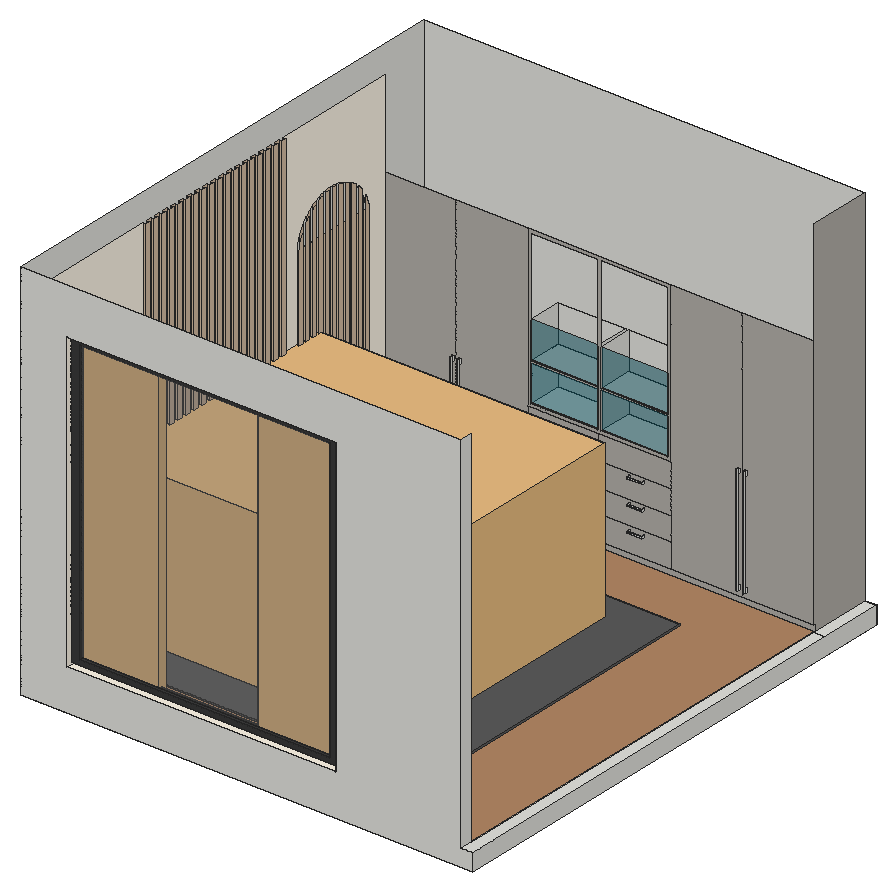
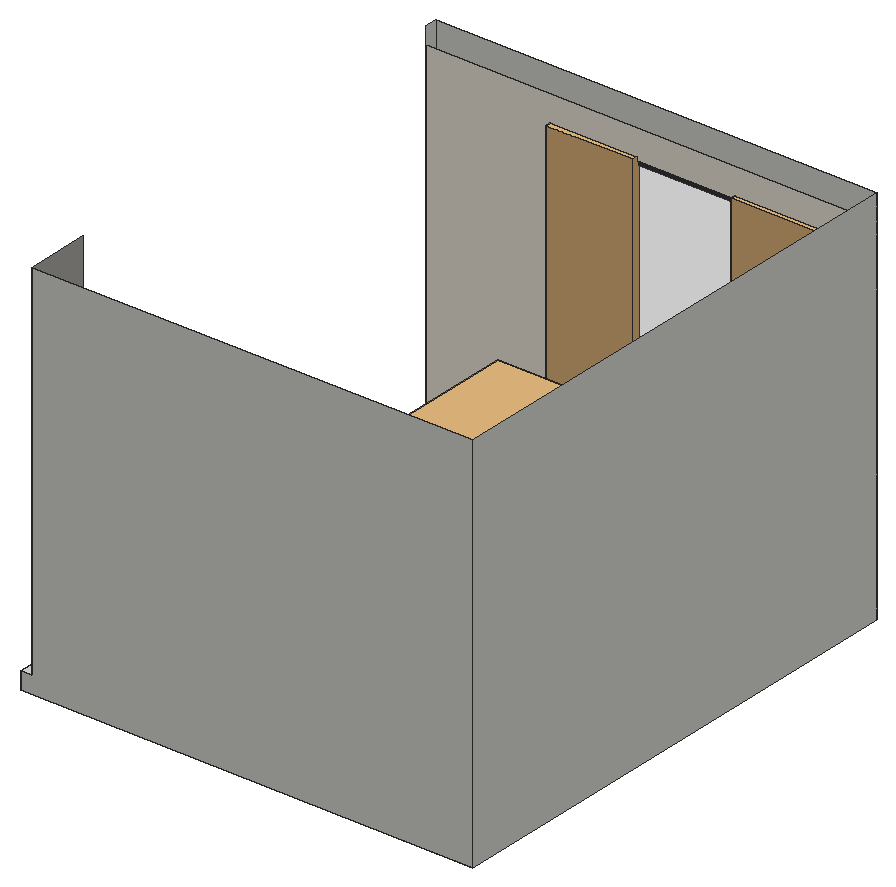
# SketchUp Ruby script. Lengths in inches.
U = 1.inch
M = Sketchup.active_model
def pt(a) = Geom::Point3d.new(a.map { |v| v * U })
def face(e, loops, mat)
  f = e.add_face(loops[0].map { |a| pt(a) })
  loops[1..].each { |l| e.add_face(l.map { |a| pt(a) }).erase! }
  f.material = f.back_material = mat if mat
  f
end
# faces: each face lists its corners as indices into pts; further lists are holes
def faces(e, pts, list, mat = nil) = list.each { |f| face(e, (f[0].is_a?(Array) ? f : [f]).map { |l| l.map { |i| pts[i] } }, mat) }
# xy, xz, yz: faces in a plane at the given z, y or x. An outline is a flat list of corners, or four numbers for a rectangle; further outlines are holes
def ring(l) = l.size == 4 ? [[l[0], l[1]], [l[2], l[1]], [l[2], l[3]], [l[0], l[3]]] : l.each_slice(2).to_a
def flat(e, list, mat, &to3) = list.each { |f| face(e, (f[0].is_a?(Array) ? f : [f]).map { |l| ring(l).map { |u, v| to3.(u, v) } }, mat) }
def xy(e, z, list, mat = nil) = flat(e, list, mat) { |x, y| [x, y, z] }
def xz(e, y, list, mat = nil) = flat(e, list, mat) { |x, z| [x, y, z] }
def yz(e, x, list, mat = nil) = flat(e, list, mat) { |y, z| [x, y, z] }
def lines(e, pts, list) = list.each { |a, b| e.add_line(pt(pts[a]), pt(pts[b])) }
# prism: a flat outline (further loops are holes) pulled along v
def prism(e, loops, v, mat = nil)
  f = face(e, loops, mat); d = Geom::Vector3d.new(v.map { |x| x * U })
  f.pushpull(f.normal.samedirection?(d) ? d.length : -d.length)
end
def box(e, o, s, mat = nil) = prism(e, [[o, [o[0] + s[0], o[1], o[2]], [o[0] + s[0], o[1] + s[1], o[2]], [o[0], o[1] + s[1], o[2]]]], [0, 0, s[2]], mat)
def at(x, y, z, deg = 0) = Geom::Transformation.translation(pt([x, y, z])) * Geom::Transformation.rotation(ORIGIN, Z_AXIS, deg.degrees)
def axes(o, x, y, z) = Geom::Transformation.new([*x, 0, *y, 0, *z, 0, *pt(o).to_a, 1])
def part(name) = M.definitions.add(name)
# library, detail: a bought-in or finely detailed component or shape, given as its bounding box
def library(name, o, s) = part(name).tap { |d| box(d.entities, o, s) }
def detail(e, o, s) = box(e.add_group.entities, o, s)
def put(e, d, t, mat = nil) = e.add_instance(d, t).tap { |i| i.material = mat if mat }
def group(e, t, mat = nil) = e.add_group.tap { |g| g.transformation = t; g.material = mat if mat }.entities
root = M.entities
M.materials.add("[0030_OldLace]").color = [253, 245, 230]
M.materials.add("[0052_FloralWhite]").color = [178, 175, 168]
M.materials.add("[Carpet Plush Charcoal]").color = [91, 91, 91]
M.materials.add("[Color M07]").color = [58, 58, 58]
M.materials.add("[Formica Laminate Light]").color = [213, 189, 164]
M.materials.add("[Sandstone]").color = [179, 135, 101]
M.materials.add("[Translucent Glass Gray]3").color = [128, 128, 128]
M.materials["[Translucent Glass Gray]3"].alpha = 0.3
M.materials.add("[Translucent Glass Tinted]").color = [3, 85, 102]
M.materials["[Translucent Glass Tinted]"].alpha = 0.48
M.materials.add("[Translucent Glass Tinted]1").color = [3, 95, 114]
M.materials["[Translucent Glass Tinted]1"].alpha = 0.48
c1 = library("Bed\#1",[-120.5625,7.36,0],[76.67,86.63,36.96])
c2 = part("POI-E1497-320-1917\#1")
xy(c2.entities,0,[[0,0,0.29,0.83],[7.21,0,7.5,0.83]])
xy(c2.entities,0.64,[[0.29,0.21,7.21,0.62]])
xy(c2.entities,0.875,[[0,0.21,7.5,0.62]])
xz(c2.entities,0.21,[[0,0.64,7.5,0.875]])
xz(c2.entities,0.62,[[0,0.64,7.5,0.875]])
yz(c2.entities,0,[[0,0,0.21,0.64,0.21,0.875,0.62,0.875,0.62,0.64,0.83,0]])
yz(c2.entities,0.29,[[0,0,0.83,0,0.62,0.64,0.21,0.64]])
yz(c2.entities,7.21,[[0,0,0.21,0.64,0.62,0.64,0.83,0]])
yz(c2.entities,7.5,[[0,0,0.83,0,0.62,0.64,0.62,0.875,0.21,0.875,0.21,0.64]])
p = [[0,0.21,0.64],[0,0,0],[0.29,0,0],[0.29,0.21,0.64],[7.21,0.21,0.64],[7.21,0,0],
  [7.5,0,0],[7.5,0.21,0.64],[0,0.83,0],[0,0.62,0.64],[0.29,0.62,0.64],[0.29,0.83,0],
  [7.5,0.83,0],[7.5,0.62,0.64],[7.21,0.62,0.64],[7.21,0.83,0]]
faces(c2.entities,p,[[0,1,2,3],[4,5,6,7],[8,9,10,11],[12,13,14,15]])
c3 = library("CURTAIN\#1",[20.4,9.88,0],[29.77,2.88,102.36])
c4 = part("WINDOW")
xy(c4.entities,0,[[0,0,59.06,1.97]],"[Color M07]")
xy(c4.entities,1.97,[[1.97,0,57.09,0.98],[1.97,0.98,57.09,1.97]],"[Color M07]")
xy(c4.entities,104.33,[[1.97,0,57.09,0.98],[1.97,0.98,57.09,1.97]],"[Color M07]")
xy(c4.entities,106.3,[[0,0,59.06,1.97]],"[Color M07]")
xz(c4.entities,0,[[[0,0,59.06,106.3],[1.97,1.97,57.09,104.33]]],"[Color M07]")
xz(c4.entities,0.98,[[1.97,1.97,57.09,104.33]],"[Translucent Glass Gray]3")
xz(c4.entities,1.97,[[[0,0,59.06,106.3],[1.97,1.97,57.09,104.33]]],"[Color M07]")
yz(c4.entities,0,[[0,0,1.97,106.3]],"[Color M07]")
yz(c4.entities,1.97,[[0,1.97,0.98,104.33],[0.98,1.97,1.97,104.33]],"[Color M07]")
yz(c4.entities,57.09,[[0,1.97,0.98,104.33],[0.98,1.97,1.97,104.33]],"[Color M07]")
yz(c4.entities,59.06,[[0,0,1.97,106.3]],"[Color M07]")
c5 = library("lamp+red",[24.48,38.48,0.35],[12.01,11.99,17.97])
xy(root,0,[[0,0,156,174]])
xy(root,5.5,[[4,4,152,4,152,153,4,153,4,144,19.91,144,19.91,143,18.91,143,18.91,132.78,121.34,132.78,121.34,20.47,18.91,20.47,18.91,13,19.91,13,19.91,12,4,12]],"[Sandstone]")
xy(root,6,[[152,0,156,152],[4,13.43,5,14.86],[4,16.29,5,17.71],[4,19.14,5,20.57],[4,22,5,23.43],
  [4,24.86,5,26.29],[4,27.71,5,29.14],[4,30.57,5,32],[4,33.43,5,34.86],[4,36.29,5,37.71],
  [4,39.14,5,40.57],[18.91,41,19.91,42],[18.91,114,19.91,115],[4,115.43,5,116.86],[4,118.29,5,119.71],
  [4,121.14,5,122.57],[4,124,5,125.43],[4,126.86,5,128.29],[4,129.71,5,131.14],[4,132.57,5,134],
  [4,135.43,5,136.86],[4,138.29,5,139.71],[4,141.14,5,142.57],[152,152,156,174]])
xy(root,6,[[4,42,18.91,42,18.91,114,4,114,4,108,5,108,5,106.29,4,106.29,4,104.57,5,104.57,5,102.86,4,102.86,4,101.14,5,101.14,5,99.43,4,99.43,4,97.71,5,97.71,5,96,4,96,4,94.29,5,94.29,5,92.57,4,92.57,4,90.86,5,90.86,5,89.14,4,89.14,4,87.43,5,87.43,5,85.71,4,85.71,4,84,5,84,5,82.29,4,82.29,4,80.57,5,80.57,5,78.86,4,78.86,4,77.14,5,77.14,5,75.43,4,75.43,4,73.71,5,73.71,5,72,4,72,4,70.29,5,70.29,5,68.57,4,68.57,4,66.86,5,66.86,5,65.14,4,65.14,4,63.43,5,63.43,5,61.71,4,61.71,4,60,5,60,5,58.29,4,58.29,4,56.57,5,56.57,5,54.86,4,54.86,4,53.14,5,53.14,5,51.43,4,51.43,4,49.71,5,49.71,5,48,4,48]],"[0030_OldLace]")
xy(root,6,[[18.91,20.47,121.34,20.47,121.34,132.78,18.91,132.78,18.91,115,19.91,115,19.91,114,18.91,114,18.91,42,19.91,42,19.91,41,18.91,41]],"[Carpet Plush Charcoal]")
xy(root,8.01,[[4,152,28.67,153],[28.67,152,53.33,153],[53.33,152,78,153],[78,152,102.67,153],[102.67,152,127.33,153],
  [127.33,152,152,153]])
xy(root,11,[[18.91,13,19.91,41],[18.91,115,19.91,143]],"[Formica Laminate Light]")
xy(root,12,[[7.91,13,19.91,41],[7.91,115,19.91,143]],"[Formica Laminate Light]")
xy(root,14.13,[[16.1875,0,108.6875,4]],"[0030_OldLace]")
xy(root,23,[[7.91,13,19.61,41],[7.91,115,19.61,143]],"[Formica Laminate Light]")
xy(root,27.91,[[19.61,23.92,20.61,27.79],[19.61,126.67,20.61,130.54]],"[Formica Laminate Light]")
xy(root,28.66,[[19.61,23.92,20.61,27.79],[19.61,126.67,20.61,130.54]],"[Formica Laminate Light]")
xy(root,29,[[19.61,13,19.91,41],[19.61,115,19.91,143]],"[Formica Laminate Light]")
xy(root,30,[[5,12,19.91,42],[5,114,19.91,144]],"[Formica Laminate Light]")
xy(root,42.24,[[54.33,152.5,77.5,164],[78.5,152.5,101.67,164]])
xy(root,42.24,[[54.33,152,77.5,152.5],[78.5,152,101.67,152.5]],"[0052_FloralWhite]")
xy(root,54.93,[[54.33,152.5,77.5,164],[78.5,152.5,101.67,164]])
xy(root,54.93,[[54.33,152,77.5,152.5],[78.5,152,101.67,152.5]],"[0052_FloralWhite]")
xy(root,55.43,[[54.33,152.5,77.5,164],[78.5,152.5,101.67,164]])
xy(root,55.43,[[54.33,152,77.5,152.5],[78.5,152,101.67,152.5]],"[0052_FloralWhite]")
xz(root,0,[[[0,0,156,0,156,6,152,6,152,132,0,132],[16.1875,14.13,108.6875,116.13]]])
xz(root,4,[[[4,5.5,152,126],[16.1875,14.13,108.6875,116.13]]],"[0030_OldLace]")
xz(root,12,[[4,5.5,5,84.25],[5,5.5,19.91,30]],"[Formica Laminate Light]")
xz(root,13,[[18.91,5.5,19.91,11],[7.91,12,19.91,23],[19.61,23,19.91,29]],"[Formica Laminate Light]")
xz(root,13.43,[[4,6,5,84.25]],"[Formica Laminate Light]")
xz(root,14.86,[[4,6,5,84.25]],"[Formica Laminate Light]")
xz(root,16.29,[[4,6,5,84.25]],"[Formica Laminate Light]")
xz(root,17.71,[[4,6,5,98.69]],"[Formica Laminate Light]")
xz(root,19.14,[[4,6,5,84.25]],"[Formica Laminate Light]")
xz(root,20.47,[[18.91,5.5,121.34,6]],"[Carpet Plush Charcoal]")
xz(root,20.57,[[4,6,5,84.25]],"[Formica Laminate Light]")
xz(root,22,[[4,6,5,84.25]],"[Formica Laminate Light]")
xz(root,23.43,[[4,6,5,84.25]],"[Formica Laminate Light]")
xz(root,23.92,[[19.61,27.91,20.61,28.66]],"[Formica Laminate Light]")
xz(root,24.86,[[4,6,5,84.25]],"[Formica Laminate Light]")
xz(root,26.29,[[4,6,5,84.25]],"[Formica Laminate Light]")
xz(root,27.71,[[4,6,5,84.25]],"[Formica Laminate Light]")
xz(root,27.79,[[19.61,27.91,20.61,28.66]],"[Formica Laminate Light]")
xz(root,29.14,[[4,6,5,84.25]],"[Formica Laminate Light]")
xz(root,30.57,[[4,6,5,84.25]],"[Formica Laminate Light]")
xz(root,32,[[4,6,5,84.25]],"[Formica Laminate Light]")
xz(root,33.43,[[4,6,5,84.25]],"[Formica Laminate Light]")
xz(root,34.86,[[4,6,5,84.25]],"[Formica Laminate Light]")
xz(root,36.29,[[4,6,5,84.25]],"[Formica Laminate Light]")
xz(root,37.71,[[4,6,5,84.25]],"[Formica Laminate Light]")
xz(root,39.14,[[4,6,5,84.25]],"[Formica Laminate Light]")
xz(root,40.57,[[4,6,5,84.25]],"[Formica Laminate Light]")
xz(root,41,[[18.91,6,19.91,11],[7.91,12,19.91,23],[19.61,23,19.91,29]],"[Formica Laminate Light]")
xz(root,42,[[4,6,5,84.25],[5,6,19.91,30]],"[Formica Laminate Light]")
xz(root,48,[[4,6,5,126]],"[Formica Laminate Light]")
xz(root,49.71,[[4,6,5,126]],"[Formica Laminate Light]")
xz(root,51.43,[[4,6,5,126]],"[Formica Laminate Light]")
xz(root,53.14,[[4,6,5,126]],"[Formica Laminate Light]")
xz(root,54.86,[[4,6,5,126]],"[Formica Laminate Light]")
xz(root,56.57,[[4,6,5,126]],"[Formica Laminate Light]")
xz(root,58.29,[[4,6,5,126]],"[Formica Laminate Light]")
xz(root,60,[[4,6,5,126]],"[Formica Laminate Light]")
xz(root,61.71,[[4,6,5,126]],"[Formica Laminate Light]")
xz(root,63.43,[[4,6,5,126]],"[Formica Laminate Light]")
xz(root,65.14,[[4,6,5,126]],"[Formica Laminate Light]")
xz(root,66.86,[[4,6,5,126]],"[Formica Laminate Light]")
xz(root,68.57,[[4,6,5,126]],"[Formica Laminate Light]")
xz(root,70.29,[[4,6,5,126]],"[Formica Laminate Light]")
xz(root,72,[[4,6,5,126]],"[Formica Laminate Light]")
xz(root,73.71,[[4,6,5,126]],"[Formica Laminate Light]")
xz(root,75.43,[[4,6,5,126]],"[Formica Laminate Light]")
xz(root,77.14,[[4,6,5,126]],"[Formica Laminate Light]")
xz(root,78.86,[[4,6,5,126]],"[Formica Laminate Light]")
xz(root,80.57,[[4,6,5,126]],"[Formica Laminate Light]")
xz(root,82.29,[[4,6,5,126]],"[Formica Laminate Light]")
xz(root,84,[[4,6,5,126]],"[Formica Laminate Light]")
xz(root,85.71,[[4,6,5,126]],"[Formica Laminate Light]")
xz(root,87.43,[[4,6,5,126]],"[Formica Laminate Light]")
xz(root,89.14,[[4,6,5,126]],"[Formica Laminate Light]")
xz(root,90.86,[[4,6,5,126]],"[Formica Laminate Light]")
xz(root,92.57,[[4,6,5,126]],"[Formica Laminate Light]")
xz(root,94.29,[[4,6,5,126]],"[Formica Laminate Light]")
xz(root,96,[[4,6,5,126]],"[Formica Laminate Light]")
xz(root,97.71,[[4,6,5,126]],"[Formica Laminate Light]")
xz(root,99.43,[[4,6,5,126]],"[Formica Laminate Light]")
xz(root,101.14,[[4,6,5,126]],"[Formica Laminate Light]")
xz(root,102.86,[[4,6,5,126]],"[Formica Laminate Light]")
xz(root,104.57,[[4,6,5,126]],"[Formica Laminate Light]")
xz(root,106.29,[[4,6,5,126]],"[Formica Laminate Light]")
xz(root,108,[[4,6,5,126]],"[Formica Laminate Light]")
xz(root,114,[[4,6,5,88.86],[5,6,19.91,30]],"[Formica Laminate Light]")
xz(root,115,[[18.91,6,19.91,11],[7.91,12,19.91,23],[19.61,23,19.91,29]],"[Formica Laminate Light]")
xz(root,115.43,[[4,6,5,88.86]],"[Formica Laminate Light]")
xz(root,116.86,[[4,6,5,88.86]],"[Formica Laminate Light]")
xz(root,118.29,[[4,6,5,88.86]],"[Formica Laminate Light]")
xz(root,119.71,[[4,6,5,88.86]],"[Formica Laminate Light]")
xz(root,121.14,[[4,6,5,88.86]],"[Formica Laminate Light]")
xz(root,122.57,[[4,6,5,88.86]],"[Formica Laminate Light]")
xz(root,124,[[4,6,5,88.86]],"[Formica Laminate Light]")
xz(root,125.43,[[4,6,5,88.86]],"[Formica Laminate Light]")
xz(root,126.67,[[19.61,27.91,20.61,28.66]],"[Formica Laminate Light]")
xz(root,126.86,[[4,6,5,88.86]],"[Formica Laminate Light]")
xz(root,128.29,[[4,6,5,88.86]],"[Formica Laminate Light]")
xz(root,129.71,[[4,6,5,88.86]],"[Formica Laminate Light]")
xz(root,130.54,[[19.61,27.91,20.61,28.66]],"[Formica Laminate Light]")
xz(root,131.14,[[4,6,5,88.86]],"[Formica Laminate Light]")
xz(root,132.57,[[4,6,5,88.86]],"[Formica Laminate Light]")
xz(root,132.78,[[18.91,5.5,121.34,6]],"[Carpet Plush Charcoal]")
xz(root,134,[[4,6,5,88.86]],"[Formica Laminate Light]")
xz(root,135.43,[[4,6,5,88.86]],"[Formica Laminate Light]")
xz(root,136.86,[[4,6,5,88.86]],"[Formica Laminate Light]")
xz(root,138.29,[[4,6,5,88.86]],"[Formica Laminate Light]")
xz(root,139.71,[[4,6,5,88.86]],"[Formica Laminate Light]")
xz(root,141.14,[[4,6,5,88.86]],"[Formica Laminate Light]")
xz(root,142.57,[[4,6,5,88.86]],"[Formica Laminate Light]")
xz(root,143,[[18.91,5.5,19.91,11],[7.91,12,19.91,23],[19.61,23,19.91,29]],"[Formica Laminate Light]")
xz(root,144,[[4,5.5,5,88.86],[5,5.5,19.91,30]],"[Formica Laminate Light]")
xz(root,152,[[4,8.01,28.67,96],[28.67,8.01,53.33,96],[53.33,8.01,78,16.32],[78,8.01,102.67,16.32],[102.67,8.01,127.33,96],
  [127.33,8.01,152,96],[53.33,16.32,78,24.625],[78,16.32,102.67,24.625],[53.33,24.625,78,32.93],[78,24.625,102.67,32.93],
  [53.33,32.93,78,41.24],[78,32.93,102.67,41.24],[[53.33,41.24,102.67,96],[54.33,42.24,77.5,95],[78.5,42.24,101.67,95]],[54.33,54.93,77.5,55.43],[78.5,54.93,101.67,55.43]],"[0052_FloralWhite]")
xz(root,152.5,[[78.5,42.24,101.67,54.93],[54.33,55.43,77.5,68.12],[78.5,55.43,101.67,68.12]],"[Translucent Glass Tinted]")
xz(root,152.5,[[54.33,42.24,77.5,54.93]],"[Translucent Glass Tinted]1")
xz(root,153,[[4,5.5,152,8.01]],"[0052_FloralWhite]")
xz(root,164,[[54.33,42.24,77.5,54.93],[78.5,42.24,101.67,54.93],[54.33,55.43,77.5,68.12],[78.5,55.43,101.67,68.12]])
xz(root,174,[[0,0,0,132,152,132,152,6,156,6,156,0]])
yz(root,0,[[0,0,174,132]])
yz(root,4,[[4,5.5,12,5.5,12,84.25,11.93,88.62,12,88.86,12.04,89.29,12.12,89.72,12.21,90.14,12.3125,90.5625,12.43,90.98,12.56,91.39,12.7,91.8,12.85,92.21,13.02,92.61,13.19,93,13.38,93.4,13.43,93.49,13.57,93.78,13.78,94.16,14,94.53,14.23,94.9,14.47,95.26,14.72,95.62,14.86,95.8,14.98,95.96,15.25,96.3,15.53,96.63,15.82,96.96,16.12,97.27,16.29,97.4375,16.42,97.58,16.74,97.87,17.0625,98.16,17.4,98.44,17.71,98.69,17.73,98.71,18.08,98.97,18.4375,99.22,18.8,99.46,19.14,99.67,19.17,99.68,19.54,99.9,19.92,100.11,20.31,100.31,21.09,100.67,21.5,100.83,21.9,100.98,22,101.01,22.3125,101.12,22.73,101.25,23.14,101.36,23.43,101.43,23.5625,101.47,23.99,101.56,24.41,101.64,24.84,101.71,24.86,101.71,25.27,101.76,26.13,101.84,26.29,101.84,26.57,101.85,27,101.86,27.43,101.85,27.71,101.84,27.87,101.84,28.73,101.76,29.14,101.71,29.16,101.71,29.59,101.64,30.01,101.56,30.4375,101.47,30.57,101.43,30.86,101.36,31.27,101.25,31.6875,101.12,32,101.01,32.1,100.98,32.5,100.83,32.91,100.67,33.69,100.31,34.08,100.11,34.46,99.9,34.83,99.68,34.86,99.67,35.2,99.46,35.5625,99.22,35.92,98.97,36.27,98.71,36.29,98.69,36.6,98.44,36.9375,98.16,37.26,97.87,37.58,97.58,37.71,97.4375,37.88,97.27,38.18,96.96,38.47,96.63,38.75,96.3,39.02,95.96,39.14,95.8,39.28,95.62,39.53,95.26,39.77,94.9,40,94.53,40.22,94.16,40.43,93.78,40.57,93.49,40.62,93.4,40.81,93,40.98,92.61,41.15,92.21,41.3,91.8,41.44,91.39,41.57,90.98,41.6875,90.5625,41.79,90.14,41.88,89.72,41.96,89.29,42,88.86,42.07,88.62,42,84.25,42,6,48,6,48,126,4,126],[144,5.5,153,5.5,153,8.01,152,8.01,152,126,108,126,108,6,114,6,114,88.86,114.04,89.29,114.12,89.72,114.21,90.14,114.3125,90.5625,114.43,90.98,114.56,91.39,114.7,91.8,114.85,92.21,115.02,92.61,115.19,93,115.38,93.4,115.43,93.49,115.57,93.78,115.78,94.16,116,94.53,116.23,94.9,116.47,95.26,116.72,95.62,116.86,95.8,116.98,95.96,117.25,96.3,117.53,96.63,117.82,96.96,118.12,97.27,118.29,97.4375,118.42,97.58,118.74,97.87,119.0625,98.16,119.4,98.44,119.71,98.69,119.73,98.71,120.08,98.97,120.4375,99.22,120.8,99.46,121.14,99.67,121.17,99.68,121.54,99.9,121.92,100.11,122.31,100.31,123.09,100.67,123.5,100.83,123.9,100.98,124,101.01,124.3125,101.12,124.73,101.25,125.14,101.36,125.43,101.43,125.5625,101.47,125.99,101.56,126.41,101.64,126.84,101.71,126.86,101.71,127.27,101.76,128.13,101.84,128.29,101.84,128.57,101.85,129,101.86,129.43,101.85,129.71,101.84,129.87,101.84,130.73,101.76,131.14,101.71,131.16,101.71,131.59,101.64,132.01,101.56,132.4375,101.47,132.57,101.43,132.86,101.36,133.27,101.25,133.6875,101.12,134,101.01,134.1,100.98,134.5,100.83,134.91,100.67,135.69,100.31,136.08,100.11,136.46,99.9,136.83,99.68,136.86,99.67,137.2,99.46,137.5625,99.22,137.92,98.97,138.27,98.71,138.29,98.69,138.6,98.44,138.9375,98.16,139.26,97.87,139.58,97.58,139.71,97.4375,139.88,97.27,140.18,96.96,140.47,96.63,140.75,96.3,141.02,95.96,141.14,95.8,141.28,95.62,141.53,95.26,141.77,94.9,142,94.53,142.22,94.16,142.43,93.78,142.57,93.49,142.62,93.4,142.81,93,142.98,92.61,143.15,92.21,143.3,91.8,143.44,91.39,143.57,90.98,143.6875,90.5625,143.79,90.14,143.88,89.72,143.96,89.29,144,88.86]],"[0030_OldLace]")
yz(root,4,[[13.43,6,14.86,6,14.86,95.8,14.72,95.62,14.47,95.26,14.23,94.9,14,94.53,13.78,94.16,13.57,93.78,13.43,93.49],[16.29,6,17.71,6,17.71,98.69,17.4,98.44,17.0625,98.16,16.74,97.87,16.42,97.58,16.29,97.4375],[19.14,6,20.57,6,20.57,100.43,20.31,100.31,19.92,100.11,19.54,99.9,19.17,99.68,19.14,99.67],[22,6,23.43,6,23.43,101.43,23.14,101.36,22.73,101.25,22.3125,101.12,22,101.01],[24.86,6,26.29,6,26.29,101.84,26.13,101.84,25.27,101.76,24.86,101.71],
  [27.71,6,29.14,6,29.14,101.71,28.73,101.76,27.87,101.84,27.71,101.84],[30.57,6,32,6,32,101.01,31.6875,101.12,31.27,101.25,30.86,101.36,30.57,101.43],[33.43,6,34.86,6,34.86,99.67,34.83,99.68,34.46,99.9,34.08,100.11,33.69,100.31,33.43,100.43],[36.29,6,37.71,6,37.71,97.4375,37.58,97.58,37.26,97.87,36.9375,98.16,36.6,98.44,36.29,98.69],[39.14,6,40.57,6,40.57,93.49,40.43,93.78,40.22,94.16,40,94.53,39.77,94.9,39.53,95.26,39.28,95.62,39.14,95.8],
  [49.71,6,51.43,126],[53.14,6,54.86,126],[56.57,6,58.29,126],[60,6,61.71,126],[63.43,6,65.14,126],
  [66.86,6,68.57,126],[70.29,6,72,126],[73.71,6,75.43,126],[77.14,6,78.86,126],[80.57,6,82.29,126],
  [84,6,85.71,126],[87.43,6,89.14,126],[90.86,6,92.57,126],[94.29,6,96,126],[97.71,6,99.43,126],
  [101.14,6,102.86,126],[104.57,6,106.29,126],[115.43,6,116.86,6,116.86,95.8,116.72,95.62,116.47,95.26,116.23,94.9,116,94.53,115.78,94.16,115.57,93.78,115.43,93.49],[118.29,6,119.71,6,119.71,98.69,119.4,98.44,119.0625,98.16,118.74,97.87,118.42,97.58,118.29,97.4375],[121.14,6,122.57,6,122.57,100.43,122.31,100.31,121.92,100.11,121.54,99.9,121.17,99.68,121.14,99.67],
  [124,6,125.43,6,125.43,101.43,125.14,101.36,124.73,101.25,124.3125,101.12,124,101.01],[126.86,6,128.29,6,128.29,101.84,128.13,101.84,127.27,101.76,126.86,101.71],[129.71,6,131.14,6,131.14,101.71,130.73,101.76,129.87,101.84,129.71,101.84],[132.57,6,134,6,134,101.01,133.6875,101.12,133.27,101.25,132.86,101.36,132.57,101.43],[135.43,6,136.86,6,136.86,99.67,136.83,99.68,136.46,99.9,136.08,100.11,135.69,100.31,135.43,100.43],
  [138.29,6,139.71,6,139.71,97.4375,139.58,97.58,139.26,97.87,138.9375,98.16,138.6,98.44,138.29,98.69],[141.14,6,142.57,6,142.57,93.49,142.43,93.78,142.22,94.16,142,94.53,141.77,94.9,141.53,95.26,141.28,95.62,141.14,95.8]],"[Formica Laminate Light]")
yz(root,5,[[13.43,6,14.86,30],[16.29,6,17.71,30],[19.14,6,20.57,30],[22,6,23.43,30],[24.86,6,26.29,30],
  [27.71,6,29.14,30],[30.57,6,32,30],[33.43,6,34.86,30],[36.29,6,37.71,30],[39.14,6,40.57,30],
  [115.43,6,116.86,30],[118.29,6,119.71,30],[121.14,6,122.57,30],[124,6,125.43,30],[126.86,6,128.29,30],
  [129.71,6,131.14,30],[132.57,6,134,30],[135.43,6,136.86,30],[138.29,6,139.71,30],[141.14,6,142.57,30]])
yz(root,5,[[48,6,49.71,126],[51.43,6,53.14,126],[54.86,6,56.57,126],[58.29,6,60,126],[61.71,6,63.43,126],
  [65.14,6,66.86,126],[68.57,6,70.29,126],[72,6,73.71,126],[75.43,6,77.14,126],[78.86,6,80.57,126],
  [82.29,6,84,126],[85.71,6,87.43,126],[89.14,6,90.86,126],[92.57,6,94.29,126],[96,6,97.71,126],
  [99.43,6,101.14,126],[102.86,6,104.57,126],[106.29,6,108,126],[12,30,13.43,30,13.43,93.49,13.38,93.4,13.19,93,13.02,92.61,12.85,92.21,12.7,91.8,12.56,91.39,12.43,90.98,12.3125,90.5625,12.21,90.14,12.12,89.72,12.04,89.29,12,88.86],[14.86,30,16.29,30,16.29,97.4375,16.12,97.27,15.82,96.96,15.53,96.63,15.25,96.3,14.98,95.96,14.86,95.8],
  [17.71,30,19.14,30,19.14,99.67,18.8,99.46,18.4375,99.22,18.08,98.97,17.73,98.71,17.71,98.69],[20.57,30,22,30,22,101.01,21.9,100.98,21.5,100.83,21.09,100.67,20.57,100.43],[23.43,30,24.86,30,24.86,101.71,24.84,101.71,24.41,101.64,23.99,101.56,23.5625,101.47,23.43,101.43],[26.29,30,27.71,30,27.71,101.84,27.43,101.85,27,101.86,26.57,101.85,26.29,101.84],[29.14,30,30.57,30,30.57,101.43,30.4375,101.47,30.01,101.56,29.59,101.64,29.16,101.71,29.14,101.71],
  [32,30,33.43,30,33.43,100.43,32.91,100.67,32.5,100.83,32.1,100.98,32,101.01],[34.86,30,36.29,30,36.29,98.69,36.27,98.71,35.92,98.97,35.5625,99.22,35.2,99.46,34.86,99.67],[37.71,30,39.14,30,39.14,95.8,39.02,95.96,38.75,96.3,38.47,96.63,38.18,96.96,37.88,97.27,37.71,97.4375],[40.57,30,42,30,42,88.86,41.96,89.29,41.88,89.72,41.79,90.14,41.6875,90.5625,41.57,90.98,41.44,91.39,41.3,91.8,41.15,92.21,40.98,92.61,40.81,93,40.62,93.4,40.57,93.49],[114,30,115.43,30,115.43,93.49,115.38,93.4,115.19,93,115.02,92.61,114.85,92.21,114.7,91.8,114.56,91.39,114.43,90.98,114.3125,90.5625,114.21,90.14,114.12,89.72,114.04,89.29,114,88.86],
  [116.86,30,118.29,30,118.29,97.4375,118.12,97.27,117.82,96.96,117.53,96.63,117.25,96.3,116.98,95.96,116.86,95.8],[119.71,30,121.14,30,121.14,99.67,120.8,99.46,120.4375,99.22,120.08,98.97,119.73,98.71,119.71,98.69],[122.57,30,124,30,124,101.01,123.9,100.98,123.5,100.83,123.09,100.67,122.57,100.43],[125.43,30,126.86,30,126.86,101.71,126.84,101.71,126.41,101.64,125.99,101.56,125.5625,101.47,125.43,101.43],[128.29,30,129.71,30,129.71,101.84,129.43,101.85,129,101.86,128.57,101.85,128.29,101.84],
  [131.14,30,132.57,30,132.57,101.43,132.4375,101.47,132.01,101.56,131.59,101.64,131.16,101.71,131.14,101.71],[134,30,135.43,30,135.43,100.43,134.91,100.67,134.5,100.83,134.1,100.98,134,101.01],[136.86,30,138.29,30,138.29,98.69,138.27,98.71,137.92,98.97,137.5625,99.22,137.2,99.46,136.86,99.67],[139.71,30,141.14,30,141.14,95.8,141.02,95.96,140.75,96.3,140.47,96.63,140.18,96.96,139.88,97.27,139.71,97.4375],[142.57,30,144,30,144,88.86,143.96,89.29,143.88,89.72,143.79,90.14,143.6875,90.5625,143.57,90.98,143.44,91.39,143.3,91.8,143.15,92.21,142.98,92.61,142.81,93,142.62,93.4,142.57,93.49]],"[Formica Laminate Light]")
yz(root,7.91,[[13,12,41,23],[115,12,143,23]],"[Formica Laminate Light]")
yz(root,16.1875,[[0,14.13,4,116.13]],"[0030_OldLace]")
yz(root,18.91,[[13,5.5,20.47,5.5,20.47,6,41,6,41,11,13,11],[132.78,5.5,143,5.5,143,11,115,11,115,6,132.78,6]],"[Formica Laminate Light]")
yz(root,19.61,[[[13,23,41,29],[23.92,27.91,27.79,28.66]],[[115,23,143,29],[126.67,27.91,130.54,28.66]]],"[Formica Laminate Light]")
yz(root,19.91,[[12,5.5,13,5.5,13,29,41,29,41,6,42,6,42,30,12,30],[143,5.5,144,5.5,144,30,114,30,114,6,115,6,115,29,143,29],[13,11,41,12],[115,11,143,12]],"[Formica Laminate Light]")
yz(root,20.61,[[23.92,27.91,27.79,28.66],[126.67,27.91,130.54,28.66]],"[Formica Laminate Light]")
yz(root,54.33,[[152.5,42.24,164,54.93],[152.5,55.43,164,68.12]])
yz(root,54.33,[[152,42.24,152.5,54.93],[152,55.43,152.5,68.12]],"[0052_FloralWhite]")
yz(root,77.5,[[152.5,42.24,164,54.93],[152.5,55.43,164,68.12]])
yz(root,77.5,[[152,42.24,152.5,54.93],[152,55.43,152.5,68.12]],"[0052_FloralWhite]")
yz(root,78.5,[[152.5,42.24,164,54.93],[152.5,55.43,164,68.12]])
yz(root,78.5,[[152,42.24,152.5,54.93],[152,55.43,152.5,68.12]],"[0052_FloralWhite]")
yz(root,101.67,[[152.5,42.24,164,54.93],[152.5,55.43,164,68.12]])
yz(root,101.67,[[152,42.24,152.5,54.93],[152,55.43,152.5,68.12]],"[0052_FloralWhite]")
yz(root,108.6875,[[0,14.13,4,116.13]],"[0030_OldLace]")
yz(root,121.34,[[20.47,5.5,132.78,6]],"[Carpet Plush Charcoal]")
yz(root,152,[[0,6,4,132]])
yz(root,152,[[4,5.5,152,6],[152,5.5,153,6]],"[0030_OldLace]")
yz(root,152,[[153,6,174,6,174,132,152,132,152,8.01,153,8.01]],"[0052_FloralWhite]")
yz(root,156,[[0,0,174,6]])
put(root,c1,axes([111.14,174.15,6],[0,1.15676,0],[-1.14,0,0],[0,0,1.45]))
put(root,c2,axes([30.3,152,10.05],[0,0,5],[-1,0,0],[0,-1,0]))
put(root,c2,axes([27.92,152,10.05],[0,0,5],[-1,0,0],[0,-1,0]))
put(root,c2,axes([128.92,152,10.05],[0,0,5],[-1,0,0],[0,-1,0]))
put(root,c2,axes([126.55,152,10.05],[0,0,5],[-1,0,0],[0,-1,0]))
put(root,c2,axes([63.47,152,14.41],[0.6888,0,0],[0,0,1],[0,-1,0]))
put(root,c2,axes([88.34,152,14.41],[0.6888,0,0],[0,0,1],[0,-1,0]))
put(root,c3,at(-4.57,-6.98,14.52))
put(root,c3,at(59.11,-6.99,14.68))
put(root,c4,axes([16.1875,1.43,15.08],[1.56633,0,0],[0,1,0],[0,0,0.95061]))
put(root,c2,axes([63.47,152,22.54],[0.6888,0,0],[0,0,1],[0,-1,0]))
put(root,c2,axes([88.34,152,22.72],[0.6888,0,0],[0,0,1],[0,-1,0]))
put(root,c5,at(-15.72,-16.64,29.66))
put(root,c5,at(-15.72,84.61,29.66))
put(root,c2,axes([63.47,152,30.79],[0.6888,0,0],[0,0,1],[0,-1,0]))
put(root,c2,axes([88.34,152,31.22],[0.6888,0,0],[0,0,1],[0,-1,0]))
